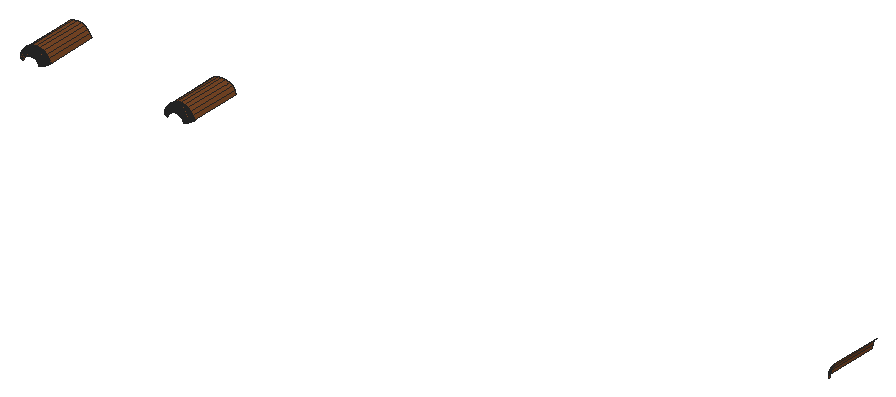
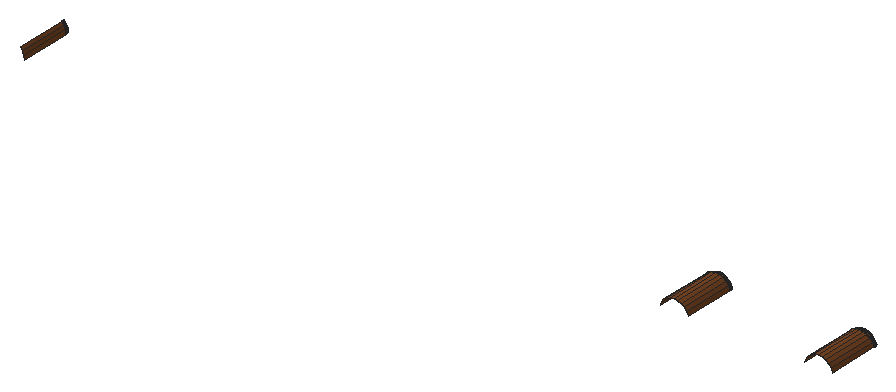
# SketchUp Ruby script. Lengths in inches.
U = 1.inch
M = Sketchup.active_model
def pt(a) = Geom::Point3d.new(a.map { |v| v * U })
def face(e, loops, mat)
  f = e.add_face(loops[0].map { |a| pt(a) })
  loops[1..].each { |l| e.add_face(l.map { |a| pt(a) }).erase! }
  f.material = f.back_material = mat if mat
  f
end
# faces: each face lists its corners as indices into pts; further lists are holes
def faces(e, pts, list, mat = nil) = list.each { |f| face(e, (f[0].is_a?(Array) ? f : [f]).map { |l| l.map { |i| pts[i] } }, mat) }
# xy, xz, yz: faces in a plane at the given z, y or x. An outline is a flat list of corners, or four numbers for a rectangle; further outlines are holes
def ring(l) = l.size == 4 ? [[l[0], l[1]], [l[2], l[1]], [l[2], l[3]], [l[0], l[3]]] : l.each_slice(2).to_a
def flat(e, list, mat, &to3) = list.each { |f| face(e, (f[0].is_a?(Array) ? f : [f]).map { |l| ring(l).map { |u, v| to3.(u, v) } }, mat) }
def xy(e, z, list, mat = nil) = flat(e, list, mat) { |x, y| [x, y, z] }
def xz(e, y, list, mat = nil) = flat(e, list, mat) { |x, z| [x, y, z] }
def yz(e, x, list, mat = nil) = flat(e, list, mat) { |y, z| [x, y, z] }
def lines(e, pts, list) = list.each { |a, b| e.add_line(pt(pts[a]), pt(pts[b])) }
# prism: a flat outline (further loops are holes) pulled along v
def prism(e, loops, v, mat = nil)
  f = face(e, loops, mat); d = Geom::Vector3d.new(v.map { |x| x * U })
  f.pushpull(f.normal.samedirection?(d) ? d.length : -d.length)
end
def box(e, o, s, mat = nil) = prism(e, [[o, [o[0] + s[0], o[1], o[2]], [o[0] + s[0], o[1] + s[1], o[2]], [o[0], o[1] + s[1], o[2]]]], [0, 0, s[2]], mat)
def at(x, y, z, deg = 0) = Geom::Transformation.translation(pt([x, y, z])) * Geom::Transformation.rotation(ORIGIN, Z_AXIS, deg.degrees)
def axes(o, x, y, z) = Geom::Transformation.new([*x, 0, *y, 0, *z, 0, *pt(o).to_a, 1])
def part(name) = M.definitions.add(name)
# library, detail: a bought-in or finely detailed component or shape, given as its bounding box
def library(name, o, s) = part(name).tap { |d| box(d.entities, o, s) }
def detail(e, o, s) = box(e.add_group.entities, o, s)
def put(e, d, t, mat = nil) = e.add_instance(d, t).tap { |i| i.material = mat if mat }
def group(e, t, mat = nil) = e.add_group.tap { |g| g.transformation = t; g.material = mat if mat }.entities
root = M.entities
M.materials.add("[Wood Veneer 01]").color = [120, 70, 37]
xz(root,0,[[27.412,33.755,27.44,33.822,27.424,33.831,27.394,33.76],[27.947,33.755,27.964,33.76,27.935,33.831,27.919,33.822],[32.404,33.757,32.433,33.826,32.418,33.834,32.387,33.762],[32.954,33.757,32.971,33.762,32.941,33.834,32.926,33.826],[27.44,33.822,27.484,33.879,27.471,33.892,27.424,33.831],
  [27.919,33.822,27.935,33.831,27.888,33.892,27.875,33.879],[32.433,33.826,32.478,33.885,32.466,33.897,32.418,33.834],[32.926,33.826,32.941,33.834,32.893,33.897,32.881,33.885],[27.484,33.879,27.541,33.923,27.532,33.939,27.471,33.892],[27.875,33.879,27.888,33.892,27.827,33.939,27.818,33.923],
  [32.478,33.885,32.537,33.93,32.528,33.945,32.466,33.897],[32.881,33.885,32.893,33.897,32.83,33.945,32.822,33.93],[27.541,33.923,27.608,33.951,27.603,33.968,27.532,33.939],[27.818,33.923,27.827,33.939,27.756,33.968,27.751,33.951],[32.537,33.93,32.606,33.958,32.601,33.975,32.528,33.945],
  [32.822,33.93,32.83,33.945,32.758,33.975,32.753,33.958],[27.608,33.951,27.679,33.96,27.679,33.978,27.603,33.968],[27.751,33.951,27.756,33.968,27.679,33.978,27.679,33.96],[32.606,33.958,32.679,33.968,32.679,33.986,32.601,33.975],[32.753,33.958,32.758,33.975,32.679,33.986,32.679,33.968]],"[Wood Veneer 01]")
p = [[55.243,0.045,33.683],[55.258,0.045,33.796],[55.249,0.054,33.799],[55.234,0.054,33.683],[55.253,0.037,33.683],[55.268,0.037,33.794],
  [55.264,0.03,33.683],[55.278,0.03,33.791],[55.276,0.024,33.683],[55.29,0.024,33.788],[55.288,0.018,33.683],[55.302,0.018,33.784],
  [55.185,0.15,33.683],[55.202,0.15,33.811],[55.2,0.165,33.812],[55.183,0.165,33.683],[55.189,0.135,33.683],[55.205,0.135,33.81],
  [55.193,0.121,33.683],[55.209,0.121,33.809],[55.198,0.108,33.683],[55.214,0.108,33.808],[55.203,0.096,33.683],[55.22,0.096,33.806],
  [55.21,0.084,33.683],[55.226,0.084,33.805],[55.217,0.073,33.683],[55.233,0.073,33.803],[55.225,0.063,33.683],[55.24,0.063,33.801],
  [55.196,2,33.813],[55.179,2,33.683],[55.179,0.216,33.683],[55.196,0.216,33.813],[55.18,0.198,33.683],[55.197,0.198,33.8125],
  [27.295,0.055,33.905],[27.25,0.055,33.798],[27.26,0.046,33.796],[27.303,0.046,33.901],[27.27,0.038,33.793],[27.312,0.038,33.895],
  [27.281,0.031,33.79],[27.322,0.031,33.89],[27.292,0.025,33.787],[27.332,0.025,33.884],[27.304,0.019,33.784],[27.343,0.019,33.877],
  [27.318,0.014,33.78],[27.355,0.014,33.871],[27.331,0.01,33.777],[27.367,0.01,33.863],[27.346,0.006,33.773],[27.38,0.006,33.856],
  [27.361,0.003,33.769],[27.394,0.003,33.848],[27.377,0.002,33.764],[27.409,0.002,33.84],[27.394,0,33.76],[27.424,0,33.831],
  [27.447,0.003,33.916],[27.435,0.006,33.927],[27.458,0.002,33.904],[27.471,0,33.892],[27.888,0,33.892],[27.935,0,33.831],
  [27.95,0.002,33.84],[27.9,0.002,33.904],[27.964,0.003,33.848],[27.912,0.003,33.916],[27.978,0.006,33.856],[27.923,0.006,33.927],
  [27.981,0.002,33.764],[27.964,0,33.76],[27.997,0.003,33.769],[28.013,0.006,33.773],[28.027,0.01,33.777],[27.991,0.01,33.863],
  [28.041,0.014,33.78],[28.004,0.014,33.871],[28.054,0.019,33.784],[28.015,0.019,33.877],[28.066,0.025,33.787],[28.026,0.025,33.884],
  [28.078,0.031,33.79],[28.037,0.031,33.89],[28.089,0.038,33.793],[28.047,0.038,33.895],[28.099,0.046,33.796],[28.056,0.046,33.901],
  [28.108,0.055,33.798],[28.064,0.055,33.905],[32.257,0.045,33.796],[32.301,0.045,33.902],[32.293,0.053,33.906],[32.248,0.053,33.799],
  [32.267,0.037,33.794],[32.31,0.037,33.897],[32.278,0.03,33.791],[32.319,0.03,33.891],[32.289,0.024,33.788],[32.329,0.024,33.885],
  [32.301,0.018,33.785],[32.34,0.018,33.879],[32.313,0.013,33.781],[32.351,0.013,33.873],[32.327,0.009,33.778],[32.363,0.009,33.866],
  [32.341,0.006,33.774],[32.376,0.006,33.859],[32.356,0.003,33.77],[32.389,0.003,33.851],[32.371,0.001,33.766],[32.403,0.001,33.843],
  [32.387,0,33.762],[32.418,0,33.834],[32.454,0.001,33.909],[32.442,0.003,33.92],[32.466,0,33.897],[32.893,0,33.897],
  [32.941,0,33.834],[32.956,0.001,33.843],[32.905,0.001,33.909],[32.97,0.003,33.851],[32.916,0.003,33.92],[32.988,0.001,33.766],
  [32.971,0,33.762],[33.003,0.003,33.77],[33.018,0.006,33.774],[32.983,0.006,33.859],[33.032,0.009,33.778],[32.995,0.009,33.866],
  [33.045,0.013,33.781],[33.007,0.013,33.873],[33.058,0.018,33.785],[33.019,0.018,33.879],[33.07,0.024,33.788],[33.029,0.024,33.885],
  [33.081,0.03,33.791],[33.039,0.03,33.891],[33.092,0.037,33.794],[33.049,0.037,33.897],[33.101,0.045,33.796],[33.058,0.045,33.902],
  [33.11,0.053,33.799],[33.066,0.053,33.906],[55.302,0.045,33.901],[55.293,0.054,33.906],[55.31,0.037,33.896],[55.32,0.03,33.891],
  [27.252,0.154,33.93],[27.202,0.154,33.811],[27.206,0.139,33.81],[27.255,0.139,33.928],[27.21,0.124,33.809],[27.258,0.124,33.926],
  [27.215,0.111,33.808],[27.263,0.111,33.924],[27.22,0.098,33.806],[27.268,0.098,33.921],[27.227,0.086,33.805],[27.273,0.086,33.918],
  [27.234,0.075,33.803],[27.28,0.075,33.914],[27.242,0.065,33.801],[27.287,0.065,33.91],[28.117,0.065,33.801],[28.072,0.065,33.91],
  [28.125,0.075,33.803],[28.079,0.075,33.914],[28.132,0.086,33.805],[28.085,0.086,33.918],[28.138,0.098,33.806],[28.091,0.098,33.921],
  [28.144,0.111,33.808],[28.096,0.111,33.924],[28.149,0.124,33.809],[28.1,0.124,33.926],[28.153,0.139,33.81],[28.104,0.139,33.928],
  [28.156,0.154,33.811],[28.107,0.154,33.93],[32.202,0.148,33.811],[32.251,0.148,33.93],[32.249,0.163,33.932],[32.2,0.163,33.812],
  [32.205,0.134,33.81],[32.254,0.134,33.929],[32.209,0.12,33.809],[32.258,0.12,33.927],[32.214,0.107,33.808],[32.262,0.107,33.924],
  [32.219,0.095,33.807],[32.267,0.095,33.921],[32.226,0.083,33.805],[32.273,0.083,33.918],[32.232,0.073,33.803],[32.279,0.073,33.915],
  [32.24,0.0625,33.801],[32.285,0.0625,33.911],[33.119,0.0625,33.801],[33.073,0.0625,33.911],[33.126,0.073,33.803],[33.08,0.073,33.915],
  [33.133,0.083,33.805],[33.086,0.083,33.918],[33.139,0.095,33.807],[33.092,0.095,33.921],[33.145,0.107,33.808],[33.096,0.107,33.924],
  [33.149,0.12,33.809],[33.101,0.12,33.927],[33.153,0.134,33.81],[33.104,0.134,33.929],[33.156,0.148,33.811],[33.107,0.148,33.93],
  [33.159,0.163,33.812],[33.109,0.163,33.932],[55.252,0.15,33.93],[55.249,0.165,33.932],[55.254,0.135,33.929],[55.258,0.121,33.927],
  [55.262,0.108,33.924],[55.267,0.096,33.921],[55.273,0.084,33.918],[55.279,0.073,33.914],[55.286,0.063,33.91],[27.246,2,33.933],
  [27.196,2,33.813],[27.196,0.221,33.813],[27.246,0.221,33.933],[27.197,0.203,33.8125],[27.247,0.203,33.933],[27.198,0.186,33.8125],
  [27.248,0.186,33.933],[27.2,0.169,33.812],[27.249,0.169,33.932],[28.159,0.169,33.812],[28.109,0.169,33.932],[28.161,0.186,33.8125],
  [28.111,0.186,33.933],[28.162,0.203,33.8125],[28.112,0.203,33.933],[28.162,0.221,33.813],[28.112,0.221,33.933],[28.162,2,33.813],
  [28.112,2,33.933],[32.246,2,33.933],[32.196,2,33.813],[32.196,0.213,33.813],[32.246,0.213,33.933],[32.197,0.196,33.8125],
  [32.247,0.196,33.933],[32.198,0.179,33.8125],[32.248,0.179,33.933],[33.161,0.179,33.8125],[33.111,0.179,33.933],[33.162,0.196,33.8125],
  [33.112,0.196,33.933],[33.162,0.213,33.813],[33.112,0.213,33.933],[33.162,2,33.813],[33.112,2,33.933],[55.246,2,33.933],
  [55.246,0.216,33.933],[55.247,0.198,33.933],[55.198,0.181,33.8125],[55.248,0.181,33.933],[27.372,0.046,33.991],[27.365,0.055,33.997],
  [27.379,0.038,33.983],[27.387,0.031,33.975],[27.396,0.025,33.967],[27.405,0.019,33.958],[27.414,0.014,33.948],[27.425,0.01,33.938],
  [27.492,0.014,34.008],[27.485,0.019,34.019],[27.499,0.01,33.995],[27.507,0.006,33.982],[27.515,0.003,33.968],[27.523,0.002,33.954],
  [27.532,0,33.939],[27.603,0,33.968],[27.598,0.002,33.985],[27.756,0,33.968],[27.827,0,33.939],[27.836,0.002,33.954],
  [27.76,0.002,33.985],[27.844,0.003,33.968],[27.852,0.006,33.982],[27.934,0.01,33.938],[27.859,0.01,33.995],[27.944,0.014,33.948],
  [27.867,0.014,34.008],[27.954,0.019,33.958],[27.873,0.019,34.019],[27.963,0.025,33.967],[27.971,0.031,33.975],[27.979,0.038,33.983],
  [27.987,0.046,33.991],[27.993,0.055,33.997],[32.37,0.045,33.992],[32.364,0.053,33.999],[32.378,0.037,33.985],[32.385,0.03,33.977],
  [32.393,0.024,33.969],[32.402,0.018,33.96],[32.411,0.013,33.951],[32.421,0.009,33.941],[32.431,0.006,33.931],[32.49,0.013,34.011],
  [32.497,0.009,33.999],[32.504,0.006,33.987],[32.512,0.003,33.974],[32.52,0.001,33.96],[32.528,0,33.945],[32.601,0,33.975],
  [32.597,0.001,33.991],[32.839,0.001,33.96],[32.762,0.001,33.991],[32.758,0,33.975],[32.83,0,33.945],[32.847,0.003,33.974],
  [32.927,0.006,33.931],[32.855,0.006,33.987],[32.9375,0.009,33.941],[32.862,0.009,33.999],[32.947,0.013,33.951],[32.869,0.013,34.011],
  [32.956,0.018,33.96],[32.965,0.024,33.969],[32.973,0.03,33.977],[32.981,0.037,33.985],[32.988,0.045,33.992],[32.995,0.053,33.999],
  [27.333,0.139,34.03],[27.33,0.154,34.032],[27.336,0.124,34.027],[27.339,0.111,34.023],[27.343,0.098,34.019],[27.348,0.086,34.015],
  [27.353,0.075,34.009],[27.359,0.065,34.004],[28,0.065,34.004],[28.005,0.075,34.009],[28.011,0.086,34.015],[28.015,0.098,34.019],
  [28.019,0.111,34.023],[28.023,0.124,34.027],[28.026,0.139,34.03],[28.028,0.154,34.032],[32.33,0.148,34.033],[32.328,0.163,34.034],
  [32.332,0.134,34.03],[32.335,0.12,34.027],[32.339,0.107,34.024],[32.343,0.095,34.02],[32.347,0.083,34.015],[32.352,0.073,34.01],
  [32.358,0.0625,34.005],[33.001,0.0625,34.005],[33.006,0.073,34.01],[33.011,0.083,34.015],[33.016,0.095,34.02],[33.02,0.107,34.024],
  [33.023,0.12,34.027],[33.026,0.134,34.03],[33.029,0.148,34.033],[33.03,0.163,34.034],[55.33,0.15,34.033],[55.328,0.165,34.034],
  [55.332,0.135,34.03],[55.335,0.121,34.027],[55.339,0.108,34.024],[27.326,2,34.037],[27.326,0.221,34.037],[27.326,0.203,34.037],
  [27.327,0.186,34.036],[27.328,0.169,34.034],[28.03,0.169,34.034],[28.032,0.186,34.036],[28.033,0.203,34.037],[28.033,0.221,34.037],
  [28.033,2,34.037],[32.326,2,34.037],[32.326,0.213,34.037],[32.326,0.196,34.037],[32.327,0.179,34.036],[33.032,0.179,34.036],
  [33.033,0.196,34.037],[33.033,0.213,34.037],[33.033,2,34.037],[55.326,2,34.037],[55.326,0.216,34.037],[55.326,0.198,34.037],
  [55.327,0.181,34.036],[27.462,0.046,34.06],[27.457,0.055,34.068],[27.467,0.038,34.051],[27.473,0.031,34.041],[27.479,0.025,34.03],
  [27.572,0.031,34.082],[27.57,0.038,34.093],[27.576,0.025,34.07],[27.579,0.019,34.058],[27.582,0.014,34.045],[27.586,0.01,34.031],
  [27.59,0.006,34.017],[27.594,0.003,34.001],[27.679,0.019,34.071],[27.679,0.014,34.058],[27.679,0.01,34.043],[27.679,0.006,34.028],
  [27.679,0.003,34.012],[27.679,0.002,33.996],[27.679,0,33.978],[27.765,0.003,34.001],[27.769,0.006,34.017],[27.773,0.01,34.031],
  [27.776,0.014,34.045],[27.78,0.019,34.058],[27.88,0.025,34.03],[27.783,0.025,34.07],[27.886,0.031,34.041],[27.786,0.031,34.082],
  [27.891,0.038,34.051],[27.789,0.038,34.093],[27.897,0.046,34.06],[27.901,0.055,34.068],[32.456,0.053,34.07],[32.461,0.045,34.062],
  [32.466,0.037,34.053],[32.471,0.03,34.043],[32.477,0.024,34.033],[32.483,0.018,34.023],[32.572,0.03,34.085],[32.569,0.037,34.095],
  [32.575,0.024,34.074],[32.578,0.018,34.062],[32.581,0.013,34.049],[32.585,0.009,34.036],[32.589,0.006,34.022],[32.593,0.003,34.007],
  [32.679,0.018,34.075],[32.679,0.013,34.062],[32.679,0.009,34.048],[32.679,0.006,34.034],[32.679,0.003,34.018],[32.679,0.001,34.002],
  [32.679,0,33.986],[32.766,0.003,34.007],[32.77,0.006,34.022],[32.774,0.009,34.036],[32.777,0.013,34.049],[32.781,0.018,34.062],
  [32.875,0.018,34.023],[32.881,0.024,34.033],[32.784,0.024,34.074],[32.887,0.03,34.043],[32.787,0.03,34.085],[32.893,0.037,34.053],
  [32.79,0.037,34.095],[32.898,0.045,34.062],[32.902,0.053,34.07],[27.434,0.139,34.108],[27.432,0.154,34.111],[27.436,0.124,34.104],
  [27.439,0.111,34.1],[27.442,0.098,34.095],[27.445,0.086,34.089],[27.449,0.075,34.083],[27.453,0.065,34.076],[27.906,0.065,34.076],
  [27.91,0.075,34.083],[27.914,0.086,34.089],[27.917,0.098,34.095],[27.92,0.111,34.1],[27.922,0.124,34.104],[27.924,0.139,34.108],
  [27.926,0.154,34.111],[32.431,0.163,34.113],[32.432,0.148,34.111],[32.434,0.134,34.108],[32.436,0.12,34.105],[32.438,0.107,34.1],
  [32.441,0.095,34.096],[32.444,0.083,34.09],[32.448,0.073,34.084],[32.452,0.0625,34.077],[32.907,0.0625,34.077],[32.911,0.073,34.084],
  [32.914,0.083,34.09],[32.917,0.095,34.096],[32.92,0.107,34.1],[32.923,0.12,34.105],[32.925,0.134,34.108],[32.926,0.148,34.111],
  [32.928,0.163,34.113],[27.429,2,34.116],[27.429,0.221,34.116],[27.43,0.203,34.116],[27.43,0.186,34.115],[27.431,0.169,34.113],
  [27.928,0.169,34.113],[27.929,0.186,34.115],[27.929,0.203,34.116],[27.929,0.221,34.116],[27.929,2,34.116],[32.429,2,34.116],
  [32.429,0.213,34.116],[32.43,0.196,34.116],[32.43,0.179,34.115],[32.929,0.179,34.115],[32.929,0.196,34.116],[32.929,0.213,34.116],
  [32.929,2,34.116],[27.567,0.046,34.103],[27.564,0.055,34.112],[27.679,0.055,34.128],[27.679,0.046,34.118],[27.679,0.038,34.107],
  [27.679,0.031,34.096],[27.679,0.025,34.084],[27.792,0.046,34.103],[27.794,0.055,34.112],[32.566,0.045,34.105],[32.564,0.053,34.114],
  [32.679,0.053,34.129],[32.679,0.045,34.12],[32.679,0.037,34.11],[32.679,0.03,34.099],[32.679,0.024,34.088],[32.792,0.045,34.105],
  [32.795,0.053,34.114],[27.552,0.139,34.157],[27.552,0.154,34.16],[27.554,0.124,34.153],[27.555,0.111,34.148],[27.556,0.098,34.142],
  [27.558,0.086,34.136],[27.56,0.075,34.129],[27.562,0.065,34.121],[27.679,0.124,34.169],[27.679,0.111,34.164],[27.679,0.098,34.159],
  [27.679,0.086,34.152],[27.679,0.075,34.145],[27.679,0.065,34.136],[27.797,0.065,34.121],[27.799,0.075,34.129],[27.801,0.086,34.136],
  [27.802,0.098,34.142],[27.804,0.111,34.148],[27.805,0.124,34.153],[27.806,0.139,34.157],[27.807,0.154,34.16],[32.551,0.148,34.16],
  [32.551,0.163,34.163],[32.552,0.134,34.157],[32.553,0.12,34.153],[32.555,0.107,34.149],[32.556,0.095,34.143],[32.558,0.083,34.137],
  [32.56,0.073,34.13],[32.562,0.0625,34.123],[32.679,0.12,34.17],[32.679,0.107,34.165],[32.679,0.095,34.159],[32.679,0.083,34.153],
  [32.679,0.073,34.146],[32.679,0.0625,34.138],[32.797,0.0625,34.123],[32.799,0.073,34.13],[32.801,0.083,34.137],[32.803,0.095,34.143],
  [32.804,0.107,34.149],[32.805,0.12,34.153],[32.806,0.134,34.157],[32.807,0.148,34.16],[32.808,0.163,34.163],[27.55,2,34.166],
  [27.55,0.221,34.166],[27.55,0.203,34.166],[27.55,0.186,34.165],[27.551,0.169,34.163],[27.808,0.169,34.163],[27.808,0.186,34.165],
  [27.809,0.203,34.166],[27.809,0.221,34.166],[27.809,2,34.166],[32.55,2,34.166],[32.55,0.213,34.166],[32.55,0.196,34.166],
  [32.55,0.179,34.165],[32.808,0.179,34.165],[32.809,0.196,34.166],[32.809,0.213,34.166],[32.809,2,34.166],[27.679,0.154,34.177],
  [27.679,0.139,34.174],[32.679,0.163,34.18],[32.679,0.148,34.177],[32.679,0.134,34.174],[27.679,2,34.183],[27.679,0.221,34.183],
  [27.679,0.203,34.183],[27.679,0.186,34.182],[27.679,0.169,34.18],[32.679,2,34.183],[32.679,0.213,34.183],[32.679,0.196,34.183],
  [32.679,0.179,34.182]]
faces(root,p,[[0,1,2,3],[4,5,1,0],[6,7,5,4],[8,9,7,6],[10,11,9,8],[12,13,14,15],[16,17,13,12],[18,19,17,16],
  [20,21,19,18],[22,23,21,20],[24,25,23,22],[26,27,25,24],[28,29,27,26],[3,2,29,28],[30,31,32,33],[34,35,33,32],
  [36,37,38,39],[39,38,40,41],[41,40,42,43],[43,42,44,45],[45,44,46,47],[47,46,48,49],[49,48,50,51],[51,50,52,53],
  [53,52,54,55],[55,54,56,57],[57,56,58,59],[55,60,61,53],[57,62,60,55],[59,63,62,57],[64,65,66,67],[67,66,68,69],
  [69,68,70,71],[72,66,65,73],[74,68,66,72],[75,70,68,74],[76,77,70,75],[78,79,77,76],[80,81,79,78],[82,83,81,80],
  [84,85,83,82],[86,87,85,84],[88,89,87,86],[90,91,89,88],[92,93,94,95],[96,97,93,92],[98,99,97,96],[100,101,99,98],
  [102,103,101,100],[104,105,103,102],[106,107,105,104],[108,109,107,106],[110,111,109,108],[112,113,111,110],[114,115,113,112],[113,116,117,111],
  [115,118,116,113],[119,120,121,122],[122,121,123,124],[125,121,120,126],[127,123,121,125],[128,129,123,127],[130,131,129,128],[132,133,131,130],
  [134,135,133,132],[136,137,135,134],[138,139,137,136],[140,141,139,138],[142,143,141,140],[144,145,143,142],[1,146,147,2],[5,148,146,1],
  [7,149,148,5],[150,151,152,153],[153,152,154,155],[155,154,156,157],[157,156,158,159],[159,158,160,161],[161,160,162,163],[163,162,164,165],
  [165,164,37,36],[166,167,91,90],[168,169,167,166],[170,171,169,168],[172,173,171,170],[174,175,173,172],[176,177,175,174],[178,179,177,176],
  [180,181,179,178],[182,183,184,185],[186,187,183,182],[188,189,187,186],[190,191,189,188],[192,193,191,190],[194,195,193,192],[196,197,195,194],
  [198,199,197,196],[95,94,199,198],[200,201,145,144],[202,203,201,200],[204,205,203,202],[206,207,205,204],[208,209,207,206],[210,211,209,208],
  [212,213,211,210],[214,215,213,212],[216,217,215,214],[13,218,219,14],[17,220,218,13],[19,221,220,17],[21,222,221,19],[23,223,222,21],
  [25,224,223,23],[27,225,224,25],[29,226,225,27],[2,147,226,29],[227,228,229,230],[230,229,231,232],[232,231,233,234],[234,233,235,236],
  [236,235,151,150],[237,238,181,180],[239,240,238,237],[241,242,240,239],[243,244,242,241],[245,246,244,243],[247,248,249,250],[251,252,250,249],
  [253,254,252,251],[185,184,254,253],[255,256,217,216],[257,258,256,255],[259,260,258,257],[261,262,260,259],[263,30,33,264],[35,265,264,33],
  [266,267,265,35],[14,219,267,266],[39,268,269,36],[41,270,268,39],[43,271,270,41],[45,272,271,43],[47,273,272,45],[49,274,273,47],
  [51,275,274,49],[53,61,275,51],[274,276,277,273],[275,278,276,274],[61,279,278,275],[60,280,279,61],[62,281,280,60],[63,282,281,62],
  [282,283,284,281],[285,286,287,288],[286,64,67,287],[287,67,69,289],[289,69,71,290],[290,71,291,292],[292,291,293,294],[294,293,295,296],
  [71,70,77,291],[291,77,79,293],[293,79,81,295],[295,81,83,297],[297,83,85,298],[298,85,87,299],[299,87,89,300],[300,89,91,301],
  [93,302,303,94],[97,304,302,93],[99,305,304,97],[101,306,305,99],[103,307,306,101],[105,308,307,103],[107,309,308,105],[109,310,309,107],
  [111,117,310,109],[311,308,309,312],[312,309,310,313],[313,310,117,314],[314,117,116,315],[315,116,118,316],[316,317,318,315],[319,320,321,322],
  [322,119,122,319],[319,122,124,323],[323,124,324,325],[325,324,326,327],[327,326,328,329],[124,123,129,324],[324,129,131,326],[326,131,133,328],
  [328,133,135,330],[330,135,137,331],[331,137,139,332],[332,139,141,333],[333,141,143,334],[334,143,145,335],[153,336,337,150],[155,338,336,153],
  [157,339,338,155],[159,340,339,157],[161,341,340,159],[163,342,341,161],[165,343,342,163],[36,269,343,165],[301,91,167,344],[344,167,169,345],
  [345,169,171,346],[346,171,173,347],[347,173,175,348],[348,175,177,349],[349,177,179,350],[350,179,181,351],[183,352,353,184],[187,354,352,183],
  [189,355,354,187],[191,356,355,189],[193,357,356,191],[195,358,357,193],[197,359,358,195],[199,360,359,197],[94,303,360,199],[335,145,201,361],
  [361,201,203,362],[362,203,205,363],[363,205,207,364],[364,207,209,365],[365,209,211,366],[366,211,213,367],[367,213,215,368],[368,215,217,369],
  [218,370,371,219],[220,372,370,218],[221,373,372,220],[222,374,373,221],[375,227,230,376],[232,377,376,230],[234,378,377,232],[236,379,378,234],
  [150,337,379,236],[351,181,238,380],[380,238,240,381],[381,240,242,382],[382,242,244,383],[246,384,383,244],[385,247,250,386],[252,387,386,250],
  [254,388,387,252],[184,353,388,254],[369,217,256,389],[389,256,258,390],[390,258,260,391],[262,392,391,260],[393,263,264,394],[265,395,394,264],
  [267,396,395,265],[219,371,396,267],[268,397,398,269],[270,399,397,268],[271,400,399,270],[272,401,400,271],[273,277,401,272],[400,402,403,399],
  [401,404,402,400],[277,405,404,401],[276,406,405,277],[278,407,406,276],[279,408,407,278],[280,409,408,279],[281,284,409,280],[410,405,406,411],
  [411,406,407,412],[412,407,408,413],[413,408,409,414],[414,409,284,415],[415,284,283,416],[416,285,288,415],[415,288,417,414],[414,417,418,413],
  [413,418,419,412],[412,419,420,411],[411,420,421,410],[288,287,289,417],[417,289,290,418],[418,290,292,419],[419,292,294,420],[420,294,296,421],
  [421,296,422,423],[423,422,424,425],[425,424,426,427],[296,295,297,422],[422,297,298,424],[424,298,299,426],[426,299,300,428],[428,300,301,429],
  [430,303,302,431],[431,302,304,432],[432,304,305,433],[433,305,306,434],[434,306,307,435],[435,307,308,311],[433,436,437,432],[434,438,436,433],
  [435,439,438,434],[311,440,439,435],[312,441,440,311],[313,442,441,312],[314,443,442,313],[315,318,443,314],[444,439,440,445],[445,440,441,446],
  [446,441,442,447],[447,442,443,448],[448,443,318,449],[449,318,317,450],[450,321,320,449],[449,320,451,448],[448,451,452,447],[447,452,453,446],
  [446,453,454,445],[445,454,455,444],[323,451,320,319],[325,452,451,323],[327,453,452,325],[329,454,453,327],[456,455,454,329],[457,458,455,456],
  [459,460,458,457],[461,462,460,459],[329,328,330,456],[456,330,331,457],[457,331,332,459],[459,332,333,461],[461,333,334,463],[463,334,335,464],
  [336,465,466,337],[338,467,465,336],[339,468,467,338],[340,469,468,339],[341,470,469,340],[342,471,470,341],[343,472,471,342],[269,398,472,343],
  [429,301,344,473],[473,344,345,474],[474,345,346,475],[475,346,347,476],[476,347,348,477],[477,348,349,478],[478,349,350,479],[479,350,351,480],
  [481,353,352,482],[482,352,354,483],[483,354,355,484],[484,355,356,485],[485,356,357,486],[486,357,358,487],[487,358,359,488],[488,359,360,489],
  [489,360,303,430],[464,335,361,490],[490,361,362,491],[491,362,363,492],[492,363,364,493],[493,364,365,494],[494,365,366,495],[495,366,367,496],
  [496,367,368,497],[497,368,369,498],[499,375,376,500],[377,501,500,376],[378,502,501,377],[379,503,502,378],[337,466,503,379],[480,351,380,504],
  [504,380,381,505],[505,381,382,506],[506,382,383,507],[384,508,507,383],[509,385,386,510],[510,386,387,511],[511,387,388,512],[512,388,353,481],
  [498,369,389,513],[513,389,390,514],[514,390,391,515],[392,516,515,391],[397,517,518,398],[399,403,517,397],[519,518,517,520],[520,517,403,521],
  [521,403,402,522],[522,402,404,523],[523,404,405,410],[410,421,423,523],[523,423,425,522],[522,425,427,521],[521,427,524,520],[520,524,525,519],
  [427,426,428,524],[524,428,429,525],[431,526,527,430],[432,437,526,431],[528,527,526,529],[529,526,437,530],[530,437,436,531],[531,436,438,532],
  [532,438,439,444],[444,455,458,532],[532,458,460,531],[531,460,462,530],[530,462,533,529],[529,533,534,528],[463,533,462,461],[464,534,533,463],
  [465,535,536,466],[467,537,535,465],[468,538,537,467],[469,539,538,468],[470,540,539,469],[471,541,540,470],[472,542,541,471],[398,518,542,472],
  [543,537,538,544],[544,538,539,545],[545,539,540,546],[546,540,541,547],[547,541,542,548],[548,542,518,519],[519,525,549,548],[548,549,550,547],
  [547,550,551,546],[546,551,552,545],[545,552,553,544],[544,553,554,543],[525,429,473,549],[549,473,474,550],[550,474,475,551],[551,475,476,552],
  [552,476,477,553],[553,477,478,554],[554,478,479,555],[555,479,480,556],[482,557,558,481],[483,559,557,482],[484,560,559,483],[485,561,560,484],
  [486,562,561,485],[487,563,562,486],[488,564,563,487],[489,565,564,488],[430,527,565,489],[566,560,561,567],[567,561,562,568],[568,562,563,569],
  [569,563,564,570],[570,564,565,571],[571,565,527,528],[528,534,572,571],[571,572,573,570],[570,573,574,569],[569,574,575,568],[568,575,576,567],
  [567,576,577,566],[490,572,534,464],[491,573,572,490],[492,574,573,491],[493,575,574,492],[494,576,575,493],[495,577,576,494],[496,578,577,495],
  [497,579,578,496],[498,580,579,497],[581,499,500,582],[501,583,582,500],[502,584,583,501],[503,585,584,502],[466,536,585,503],[556,480,504,586],
  [586,504,505,587],[587,505,506,588],[588,506,507,589],[508,590,589,507],[591,509,510,592],[511,593,592,510],[512,594,593,511],[481,558,594,512],
  [513,595,580,498],[514,596,595,513],[515,597,596,514],[516,598,597,515],[599,536,535,600],[600,535,537,543],[543,554,555,600],[600,555,556,599],
  [601,558,557,602],[602,557,559,603],[603,559,560,566],[566,577,578,603],[603,578,579,602],[602,579,580,601],[604,581,582,605],[605,582,583,606],
  [606,583,584,607],[607,584,585,608],[608,585,536,599],[599,556,586,608],[608,586,587,607],[607,587,588,606],[606,588,589,605],[590,604,605,589],
  [609,591,592,610],[610,592,593,611],[611,593,594,612],[612,594,558,601],[601,580,595,612],[612,595,596,611],[611,596,597,610],[598,609,610,597]],"[Wood Veneer 01]")
